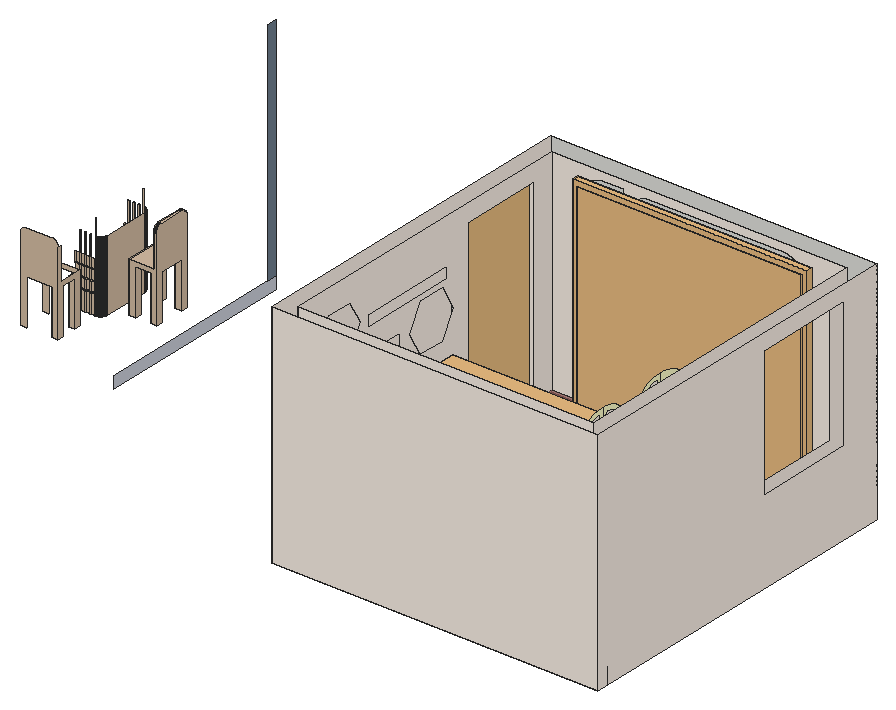
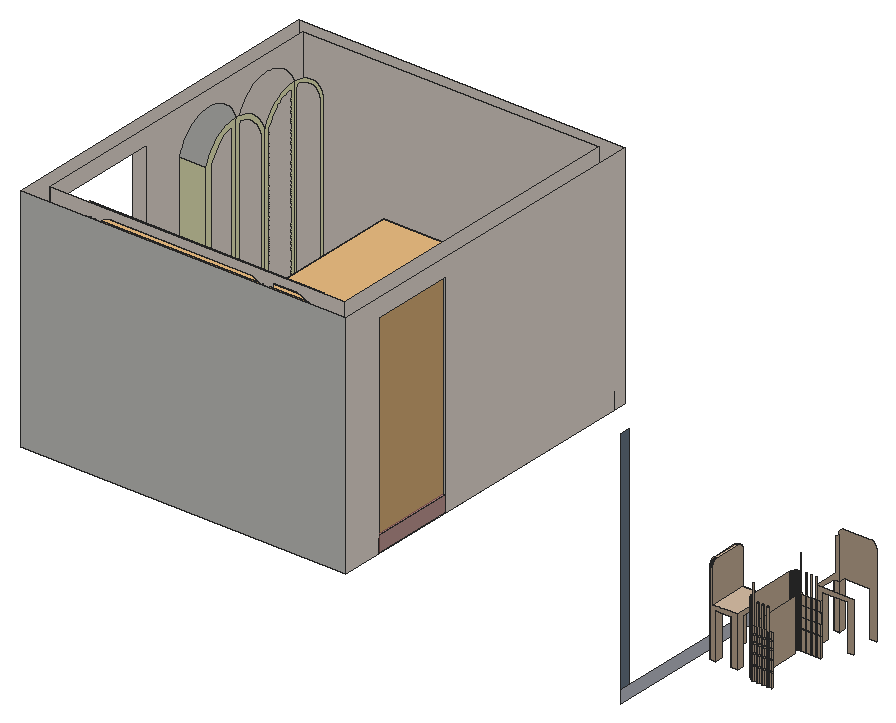
# SketchUp Ruby script. Lengths in inches.
U = 1.inch
M = Sketchup.active_model
def pt(a) = Geom::Point3d.new(a.map { |v| v * U })
def face(e, loops, mat)
  f = e.add_face(loops[0].map { |a| pt(a) })
  loops[1..].each { |l| e.add_face(l.map { |a| pt(a) }).erase! }
  f.material = f.back_material = mat if mat
  f
end
# faces: each face lists its corners as indices into pts; further lists are holes
def faces(e, pts, list, mat = nil) = list.each { |f| face(e, (f[0].is_a?(Array) ? f : [f]).map { |l| l.map { |i| pts[i] } }, mat) }
# xy, xz, yz: faces in a plane at the given z, y or x. An outline is a flat list of corners, or four numbers for a rectangle; further outlines are holes
def ring(l) = l.size == 4 ? [[l[0], l[1]], [l[2], l[1]], [l[2], l[3]], [l[0], l[3]]] : l.each_slice(2).to_a
def flat(e, list, mat, &to3) = list.each { |f| face(e, (f[0].is_a?(Array) ? f : [f]).map { |l| ring(l).map { |u, v| to3.(u, v) } }, mat) }
def xy(e, z, list, mat = nil) = flat(e, list, mat) { |x, y| [x, y, z] }
def xz(e, y, list, mat = nil) = flat(e, list, mat) { |x, z| [x, y, z] }
def yz(e, x, list, mat = nil) = flat(e, list, mat) { |y, z| [x, y, z] }
def lines(e, pts, list) = list.each { |a, b| e.add_line(pt(pts[a]), pt(pts[b])) }
# prism: a flat outline (further loops are holes) pulled along v
def prism(e, loops, v, mat = nil)
  f = face(e, loops, mat); d = Geom::Vector3d.new(v.map { |x| x * U })
  f.pushpull(f.normal.samedirection?(d) ? d.length : -d.length)
end
def box(e, o, s, mat = nil) = prism(e, [[o, [o[0] + s[0], o[1], o[2]], [o[0] + s[0], o[1] + s[1], o[2]], [o[0], o[1] + s[1], o[2]]]], [0, 0, s[2]], mat)
def at(x, y, z, deg = 0) = Geom::Transformation.translation(pt([x, y, z])) * Geom::Transformation.rotation(ORIGIN, Z_AXIS, deg.degrees)
def axes(o, x, y, z) = Geom::Transformation.new([*x, 0, *y, 0, *z, 0, *pt(o).to_a, 1])
def part(name) = M.definitions.add(name)
# library, detail: a bought-in or finely detailed component or shape, given as its bounding box
def library(name, o, s) = part(name).tap { |d| box(d.entities, o, s) }
def detail(e, o, s) = box(e.add_group.entities, o, s)
def put(e, d, t, mat = nil) = e.add_instance(d, t).tap { |i| i.material = mat if mat }
def group(e, t, mat = nil) = e.add_group.tap { |g| g.transformation = t; g.material = mat if mat }.entities
root = M.entities
M.materials.add("[0009_Linen]").color = [250, 240, 230]
M.materials.add("[0111_SlateGray]").color = [112, 128, 144]
M.materials.add("[Color E01]").color = [255, 255, 204]
M.materials.add("[Formica Laminate Light]").color = [213, 189, 164]
M.materials.add("[Marble Carrara Floor Tile]").color = [204, 208, 219]
M.materials.add("[Wood Square Tile 02]").color = [160, 101, 97]
M.materials["[Wood Square Tile 02]"].alpha = 0.73
c1 = library("1000x2100 L\#1",[0,0,0],[39.37,8.78,82.68])
c2 = library("Untitled+(2)",[-25.65,-58.99,0],[75.48,89.46,37.24])
xy(root,0,[[518.64,0,702.89,197]])
xy(root,0,[[315.45,97.95,319.1,101.59],[309.81,124.79,310.17,125.33],[312.73,124.79,313.09,125.33],[315.65,124.79,316.01,125.33],[318.58,124.79,318.9375,125.33],
  [309.52,159.08,310.35,159.77],[312.38,159.08,313.21,159.77],[315.25,159.08,316.07,159.77],[318.11,159.08,318.9375,159.77]],"[Formica Laminate Light]")
xy(root,7.64,[[307.48,159.08,309.52,159.77],[310.35,159.08,312.38,159.77],[313.21,159.08,315.25,159.77],[316.07,159.08,318.11,159.77]],"[Formica Laminate Light]")
xy(root,8.44,[[307.48,159.08,309.52,159.77],[310.35,159.08,312.38,159.77],[313.21,159.08,315.25,159.77],[316.07,159.08,318.11,159.77]],"[Formica Laminate Light]")
xy(root,9.25,[[527.89,6.9375,695.01,6.9375,695.01,12.1875,679.64,12.1875,679.64,94.5625,695.01,94.5625,695.01,185.9375,677.76,185.9375,677.76,179.1875,545.7,179.1875,545.7,185.9375,527.89,185.9375,527.89,173.6875,518.64,173.6875,518.64,126.5625,527.89,126.5625]],"[Wood Square Tile 02]")
xy(root,11.02,[[307.24,124.79,309.81,125.33],[310.17,124.79,312.73,125.33],[313.09,124.79,315.65,125.33],[316.01,124.79,318.58,125.33]],"[Formica Laminate Light]")
xy(root,11.55,[[307.24,124.79,309.81,125.33],[310.17,124.79,312.73,125.33],[313.09,124.79,315.65,125.33],[316.01,124.79,318.58,125.33]],"[Formica Laminate Light]")
xy(root,13.77,[[307.48,159.08,309.52,159.77],[310.35,159.08,312.38,159.77],[313.21,159.08,315.25,159.77],[316.07,159.08,318.11,159.77]],"[Formica Laminate Light]")
xy(root,14.57,[[307.48,159.08,309.52,159.77],[310.35,159.08,312.38,159.77],[313.21,159.08,315.25,159.77],[316.07,159.08,318.11,159.77]],"[Formica Laminate Light]")
xy(root,17.15,[[307.24,124.79,309.81,125.33],[310.17,124.79,312.73,125.33],[313.09,124.79,315.65,125.33],[316.01,124.79,318.58,125.33]],"[Formica Laminate Light]")
xy(root,19.01,[[307.48,159.08,309.52,159.77],[310.35,159.08,312.38,159.77],[313.21,159.08,315.25,159.77],[316.07,159.08,318.11,159.77]],"[Formica Laminate Light]")
xy(root,19.8125,[[307.48,159.08,309.52,159.77],[310.35,159.08,312.38,159.77],[313.21,159.08,315.25,159.77],[316.07,159.08,318.11,159.77]],"[Formica Laminate Light]")
xy(root,23.36,[[307.24,124.79,309.81,125.33],[310.17,124.79,312.73,125.33],[313.09,124.79,315.65,125.33],[316.01,124.79,318.58,125.33]],"[Formica Laminate Light]")
xy(root,23.54,[[307.48,159.08,309.52,159.77],[310.35,159.08,312.38,159.77],[313.21,159.08,315.25,159.77],[316.07,159.08,318.11,159.77]],"[Formica Laminate Light]")
xy(root,24.34,[[307.48,159.08,309.52,159.77],[310.35,159.08,312.38,159.77],[313.21,159.08,315.25,159.77],[316.07,159.08,318.11,159.77]],"[Formica Laminate Light]")
xy(root,28.25,[[329.76,134.98,343.65,156.18]],"[Formica Laminate Light]")
xy(root,50.4375,[[343.65,138.2,345.53,152.74]],"[Formica Laminate Light]")
xz(root,0,[[518.64,0,702.89,129.75]],"[0009_Linen]")
xz(root,6.9375,[[527.89,9.25,695.01,129.75]],"[0009_Linen]")
xz(root,12.1875,[[679.64,9.25,695.01,104.7]],"[Color E01]")
xz(root,53.375,[[679.64,9.25,695.01,104.7]])
xz(root,94.5625,[[679.64,9.25,695.01,104.7]],"[Color E01]")
xz(root,97.95,[[297.89,0,301.53,0,301.53,25.5625,315.45,25.5625,315.45,0,319.1,0,319.1,46.82,319.09,47.28,319.02,47.74,318.89,48.1875,318.7,48.61,318.45,49.01,318.15,49.37,317.8125,49.68,317.43,49.95,317.02,50.16,316.58,50.3125,316.125,50.41,315.66,50.4375,301.11,50.4375,300.68,50.36,300.26,50.23,299.85,50.05,299.47,49.82,299.125,49.55,298.8125,49.24,298.54,48.89,298.3125,48.52,298.13,48.12,298,47.69,297.92,47.26,297.89,46.82]],"[Formica Laminate Light]")
xz(root,101.59,[[315.45,0,319.1,25.5625]],"[Formica Laminate Light]")
xz(root,110.07,[[315.45,0,319.1,25.5625]],"[Formica Laminate Light]")
xz(root,113.72,[[297.89,0,297.89,28.25,319.1,28.25,319.1,0,315.45,0,315.45,25.5625,301.35,25.5625,301.35,0]],"[Formica Laminate Light]")
xz(root,124.79,[[309.81,0,310.17,40.33],[312.73,0,313.09,40.33],[315.65,0,316.01,40.33],[307.24,11.02,309.81,11.55],[310.17,11.02,312.73,11.55],
  [313.09,11.02,315.65,11.55],[316.01,11.02,318.58,11.55],[307.24,17.15,309.81,17.68],[310.17,17.15,312.73,17.68],[313.09,17.15,315.65,17.68],
  [316.01,17.15,318.58,17.68],[307.24,23.36,309.81,23.9],[310.17,23.36,312.73,23.9],[313.09,23.36,315.65,23.9],[316.01,23.36,318.58,23.9]],"[Formica Laminate Light]")
xz(root,125.33,[[307.24,0,309.81,11.02],[309.81,0,310.17,11.02],[310.17,0,312.73,11.02],[312.73,0,313.09,11.02],[313.09,0,315.65,11.02],
  [315.65,0,316.01,11.02],[316.01,0,318.58,11.02],[318.58,0,318.58,11.02,316.01,11.02,316.01,11.55,318.58,11.55,318.58,49.31,318.9375,49.31,318.9375,0],[309.81,11.02,310.17,11.55],[312.73,11.02,313.09,11.55],
  [315.65,11.02,316.01,11.55],[307.24,11.55,309.81,17.15],[309.81,11.55,310.17,40.33],[310.17,11.55,312.73,17.15],[312.73,11.55,313.09,40.33],
  [313.09,11.55,315.65,17.15],[315.65,11.55,316.01,40.33],[316.01,11.55,318.58,17.15],[307.24,17.15,309.81,23.36],[310.17,17.15,312.73,23.36],
  [313.09,17.15,315.65,23.36],[316.01,17.15,318.58,23.36],[307.24,23.36,309.81,28.96],[310.17,23.36,312.73,28.96],[313.09,23.36,315.65,28.96],
  [316.01,23.36,318.58,28.96]],"[Formica Laminate Light]")
xz(root,126.5625,[[518.64,9.25,527.89,119.9375]])
xz(root,134.98,[[329.76,0,333.4,0,333.4,25.5625,341.88,25.5625,341.88,0,345.53,0,345.53,46.82,343.65,46.82,343.65,28.25,329.76,28.25]],"[Formica Laminate Light]")
xz(root,138.43,[[329.76,0,333.4,25.5625]],"[Formica Laminate Light]")
xz(root,138.62,[[341.88,0,345.53,25.5625]],"[Formica Laminate Light]")
xz(root,152.54,[[329.76,0,333.4,25.5625],[341.88,0,345.53,25.5625]],"[Formica Laminate Light]")
xz(root,156.18,[[329.76,0,329.76,28.25,343.65,28.25,343.65,46.82,345.53,46.82,345.53,0,341.88,0,341.88,25.5625,333.4,25.5625,333.4,0]],"[Formica Laminate Light]")
xz(root,159.08,[[307.48,0,309.52,7.64],[309.52,0,310.35,40.33],[310.35,0,312.38,7.64],[312.38,0,313.21,40.33],[313.21,0,315.25,7.64],
  [315.25,0,316.07,40.33],[316.07,0,318.11,7.64],[318.11,0,318.9375,0,318.9375,49.31,318.11,49.31,318.11,8.44,316.07,8.44,316.07,7.64,318.11,7.64],[307.48,8.44,309.52,13.77],[310.35,8.44,312.38,13.77],
  [313.21,8.44,315.25,13.77],[316.07,8.44,318.11,13.77],[307.48,13.77,309.52,14.57],[310.35,13.77,312.38,14.57],[313.21,13.77,315.25,14.57],
  [316.07,13.77,318.11,14.57],[307.48,14.57,309.52,19.01],[310.35,14.57,312.38,19.01],[313.21,14.57,315.25,19.01],[316.07,14.57,318.11,19.01],
  [307.48,19.01,309.52,19.8125],[310.35,19.01,312.38,19.8125],[313.21,19.01,315.25,19.8125],[316.07,19.01,318.11,19.8125],[307.48,19.8125,309.52,23.54],
  [310.35,19.8125,312.38,23.54],[313.21,19.8125,315.25,23.54],[316.07,19.8125,318.11,23.54],[307.48,23.54,309.52,24.34],[310.35,23.54,312.38,24.34],
  [313.21,23.54,315.25,24.34],[316.07,23.54,318.11,24.34],[307.48,24.34,309.52,27.9],[310.35,24.34,312.38,27.9],[313.21,24.34,315.25,27.9],
  [316.07,24.34,318.11,27.9]],"[Formica Laminate Light]")
xz(root,159.77,[[309.52,0,310.35,40.33],[312.38,0,313.21,40.33],[315.25,0,316.07,40.33],[307.48,7.64,309.52,8.44],[310.35,7.64,312.38,8.44],
  [313.21,7.64,315.25,8.44],[316.07,7.64,318.11,8.44],[307.48,13.77,309.52,14.57],[310.35,13.77,312.38,14.57],[313.21,13.77,315.25,14.57],
  [316.07,13.77,318.11,14.57],[307.48,19.01,309.52,19.8125],[310.35,19.01,312.38,19.8125],[313.21,19.01,315.25,19.8125],[316.07,19.01,318.11,19.8125],
  [307.48,23.54,309.52,24.34],[310.35,23.54,312.38,24.34],[313.21,23.54,315.25,24.34],[316.07,23.54,318.11,24.34]],"[Formica Laminate Light]")
xz(root,173.6875,[[518.64,9.25,527.89,119.9375]],"[0009_Linen]")
xz(root,185.9375,[[[527.89,9.25,545.7,9.25,545.7,113.87,545.78,115.23,546.02,116.58,546.42,117.89,546.97,119.14,547.66,120.32,548.49,121.41,549.4375,122.39,550.5,123.25,551.65,123.99,552.89,124.58,554.18,125.02,555.52,125.3125,569.01,125.3125,569.01,47.68,569.08,46.64,569.28,45.61,569.62,44.62,570.08,43.68,570.66,42.8125,571.35,42.03,572.14,41.34,573.01,40.76,573.94,40.3,574.93,39.96,575.96,39.76,577,39.6875,659.67,39.6875,662.04,39.53,664.36,39.07,666.6,38.3125,668.72,37.26,670.68,35.95,672.46,34.39,674.02,32.61,675.34,30.64,676.38,28.52,677.14,26.28,677.61,23.96,677.76,21.6,677.76,9.25,695.01,9.25,695.01,129.75,527.89,129.75],[582.21,45.28,581.02,45.62,579.875,46.08,578.79,46.66,577.78,47.37,576.86,48.18,576.04,49.08,575.34,50.07,574.75,51.14,574.3,52.26,573.98,53.42,573.79,54.61,573.75,55.82,573.75,116.08,573.82,117.21,574.03,118.3125,574.375,119.39,574.85,120.41,575.46,121.375,576.17,122.26,576.99,123.05,577.91,123.75,578.9,124.33,579.96,124.78,581.07,125.11,582.21,125.3125,659.93,125.3125,661.12,125.23,662.29,124.99,663.4,124.58,664.45,124.03,665.41,123.34,666.25,122.53,666.97,121.61,667.55,120.6,667.97,119.52,668.24,118.39,668.26,118.12,668.33,117.24,668.26,116.08,668.26,55.82,668.19,54.63,667.99,53.46,667.66,52.3125,667.21,51.21,666.63,50.16,665.9375,49.18,665.14,48.28,664.25,47.46,663.27,46.75,662.21,46.14,661.1,45.65,659.93,45.28]]],"[0009_Linen]")
xz(root,197,[[518.64,0,702.89,129.75]])
yz(root,307.24,[[124.79,0,125.33,11.02],[124.79,11.02,125.33,11.55],[124.79,11.55,125.33,17.15],[124.79,23.36,125.33,28.96]],"[Formica Laminate Light]")
yz(root,307.48,[[159.08,0,159.77,7.64],[159.08,7.64,159.77,8.44],[159.08,8.44,159.77,13.77],[159.08,13.77,159.77,14.57],[159.08,14.57,159.77,19.01],
  [159.08,19.01,159.77,19.8125],[159.08,19.8125,159.77,23.54],[159.08,23.54,159.77,24.34],[159.08,24.34,159.77,27.9]],"[Formica Laminate Light]")
yz(root,309.52,[[159.08,0,159.77,7.64],[159.08,7.64,159.77,8.44],[159.08,8.44,159.77,13.77],[159.08,13.77,159.77,14.57],[159.08,14.57,159.77,19.01],
  [159.08,19.01,159.77,19.8125],[159.08,19.8125,159.77,23.54],[159.08,23.54,159.77,24.34],[159.08,24.34,159.77,27.9]],"[Formica Laminate Light]")
yz(root,309.81,[[124.79,0,125.33,11.02],[124.79,11.02,125.33,11.55],[124.79,11.55,125.33,17.15],[124.79,17.15,125.33,23.36],[124.79,23.36,125.33,28.96]],"[Formica Laminate Light]")
yz(root,310.17,[[124.79,0,125.33,11.02],[124.79,11.02,125.33,11.55],[124.79,11.55,125.33,17.15],[124.79,17.15,125.33,23.36],[124.79,23.36,125.33,28.96]],"[Formica Laminate Light]")
yz(root,310.35,[[159.08,0,159.77,7.64],[159.08,7.64,159.77,8.44],[159.08,8.44,159.77,13.77],[159.08,13.77,159.77,14.57],[159.08,14.57,159.77,19.01],
  [159.08,19.01,159.77,19.8125],[159.08,19.8125,159.77,23.54],[159.08,23.54,159.77,24.34],[159.08,24.34,159.77,27.9]],"[Formica Laminate Light]")
yz(root,312.38,[[159.08,0,159.77,7.64],[159.08,7.64,159.77,8.44],[159.08,8.44,159.77,13.77],[159.08,13.77,159.77,14.57],[159.08,14.57,159.77,19.01],
  [159.08,19.01,159.77,19.8125],[159.08,19.8125,159.77,23.54],[159.08,23.54,159.77,24.34],[159.08,24.34,159.77,27.9]],"[Formica Laminate Light]")
yz(root,312.73,[[124.79,0,125.33,11.02],[124.79,11.02,125.33,11.55],[124.79,11.55,125.33,17.15],[124.79,17.15,125.33,23.36],[124.79,23.36,125.33,28.96]],"[Formica Laminate Light]")
yz(root,313.09,[[124.79,0,125.33,11.02],[124.79,11.02,125.33,11.55],[124.79,11.55,125.33,17.15],[124.79,17.15,125.33,23.36],[124.79,23.36,125.33,28.96]],"[Formica Laminate Light]")
yz(root,313.21,[[159.08,0,159.77,7.64],[159.08,7.64,159.77,8.44],[159.08,8.44,159.77,13.77],[159.08,13.77,159.77,14.57],[159.08,14.57,159.77,19.01],
  [159.08,19.01,159.77,19.8125],[159.08,19.8125,159.77,23.54],[159.08,23.54,159.77,24.34],[159.08,24.34,159.77,27.9]],"[Formica Laminate Light]")
yz(root,315.25,[[159.08,0,159.77,7.64],[159.08,7.64,159.77,8.44],[159.08,8.44,159.77,13.77],[159.08,13.77,159.77,14.57],[159.08,14.57,159.77,19.01],
  [159.08,19.01,159.77,19.8125],[159.08,19.8125,159.77,23.54],[159.08,23.54,159.77,24.34],[159.08,24.34,159.77,27.9]],"[Formica Laminate Light]")
yz(root,315.45,[[97.95,0,101.59,25.5625],[110.07,0,113.72,25.5625]],"[Formica Laminate Light]")
yz(root,315.65,[[124.79,0,125.33,11.02],[124.79,11.02,125.33,11.55],[124.79,11.55,125.33,17.15],[124.79,17.15,125.33,23.36],[124.79,23.36,125.33,28.96]],"[Formica Laminate Light]")
yz(root,316.01,[[124.79,0,125.33,11.02],[124.79,11.02,125.33,11.55],[124.79,11.55,125.33,17.15],[124.79,17.15,125.33,23.36],[124.79,23.36,125.33,28.96]],"[Formica Laminate Light]")
yz(root,316.07,[[159.08,0,159.77,7.64],[159.08,7.64,159.77,8.44],[159.08,8.44,159.77,13.77],[159.08,13.77,159.77,14.57],[159.08,14.57,159.77,19.01],
  [159.08,19.01,159.77,19.8125],[159.08,19.8125,159.77,23.54],[159.08,23.54,159.77,24.34],[159.08,24.34,159.77,27.9]],"[Formica Laminate Light]")
yz(root,318.11,[[159.08,0,159.77,7.64],[159.08,8.44,159.77,13.77],[159.08,13.77,159.77,14.57],[159.08,14.57,159.77,19.01],[159.08,19.01,159.77,19.8125],
  [159.08,19.8125,159.77,23.54],[159.08,23.54,159.77,24.34],[159.08,24.34,159.77,27.9]],"[Formica Laminate Light]")
yz(root,318.58,[[124.79,0,125.33,11.02],[124.79,11.55,125.33,17.15],[124.79,17.15,125.33,23.36],[124.79,23.36,125.33,28.96]],"[Formica Laminate Light]")
yz(root,318.9375,[[128.96,0,155.08,28.69]],"[Formica Laminate Light]")
yz(root,319.1,[[97.95,0,101.59,0,101.59,25.5625,110.07,25.5625,110.07,0,113.72,0,113.72,28.25,99.82,28.25,99.82,46.82,97.95,46.82]],"[Formica Laminate Light]")
yz(root,322.35,[[128.96,0,155.08,40.33]],"[Formica Laminate Light]")
yz(root,329.76,[[134.98,0,134.98,28.25,156.18,28.25,156.18,0,152.54,0,152.54,25.5625,138.43,25.5625,138.43,0]],"[Formica Laminate Light]")
yz(root,333.4,[[134.98,0,138.43,25.5625],[152.54,0,156.18,25.5625]],"[Formica Laminate Light]")
yz(root,341.88,[[134.98,0,138.62,25.5625],[152.54,0,156.18,25.5625]],"[Formica Laminate Light]")
yz(root,343.65,[[134.98,28.25,134.98,46.82,135,47.26,135.08,47.69,135.21,48.12,135.4,48.52,135.625,48.89,135.9,49.24,136.21,49.55,136.56,49.82,136.9375,50.05,137.34,50.23,137.76,50.36,138.2,50.4375,152.74,50.4375,153.21,50.41,153.66,50.3125,154.1,50.16,154.52,49.95,154.9,49.68,155.24,49.37,155.54,49.01,155.78,48.61,155.97,48.1875,156.1,47.74,156.17,47.28,156.18,46.82,156.18,28.25]],"[Formica Laminate Light]")
yz(root,345.53,[[134.98,0,138.62,0,138.62,25.5625,152.54,25.5625,152.54,0,156.18,0,156.18,46.82,156.17,47.28,156.1,47.74,155.97,48.1875,155.78,48.61,155.54,49.01,155.24,49.37,154.9,49.68,154.52,49.95,154.1,50.16,153.66,50.3125,153.21,50.41,152.74,50.4375,138.2,50.4375,137.76,50.36,137.34,50.23,136.9375,50.05,136.56,49.82,136.21,49.55,135.9,49.24,135.625,48.89,135.4,48.52,135.21,48.12,135.08,47.69,135,47.26,134.98,46.82]],"[Formica Laminate Light]")
yz(root,358.53,[[197,0,202.625,129.75]],"[0111_SlateGray]")
yz(root,358.53,[[88,-6.9375,202.625,0]],"[Marble Carrara Floor Tile]")
yz(root,518.64,[[0,0,0,129.75,197,129.75,197,0,173.6875,0,173.6875,119.9375,126.5625,119.9375,126.5625,0]],"[0009_Linen]")
yz(root,518.64,[[126.5625,0,173.6875,9.25]],"[Wood Square Tile 02]")
yz(root,527.89,[[[6.9375,9.25,126.5625,9.25,126.5625,119.9375,173.6875,119.9375,173.6875,9.25,185.9375,9.25,185.9375,129.75,6.9375,129.75],[93.09,67.64,85.1875,81.33,93.09,95.02,108.9,95.02,116.8,81.33,108.9,67.64],[28.21,89.72,20.6,102.9,28.21,116.09,43.44,116.09,51.05,102.9,43.44,89.72],[24.59,78.19,78.67,85.38],[56.41,97.75,112.29,104.19]]],"[0009_Linen]")
yz(root,545.7,[[182.5625,9.25,185.9375,106.81]],"[Color E01]")
yz(root,677.76,[[182.5625,9.25,185.9375,21.6]],"[Color E01]")
yz(root,679.64,[[14.26,11.32,14.26,104.4,14.79,106.23,15.6,108.15,16.62,109.97,17.83,111.66,19.22,113.21,20.78,114.59,22.49,115.79,24.3125,116.8,26.24,117.59,28.24,118.16,30.29,118.51,30.29,11.32],[35.13,12.02,35.13,117.7,36.47,117.48,38.45,116.93,40.37,116.16,42.1875,115.19,43.89,114.04,45.46,112.7,46.88,111.2,48.12,109.56,49.18,107.79,50.04,105.92,50.6,104.25,50.6,12.02],[56.16,12.03,56.16,104.3,56.65,105.99,57.43,107.83,58.41,109.58,59.57,111.21,60.91,112.7,62.41,114.03,64.05,115.1875,65.81,116.15,67.66,116.92,69.59,117.47,70.78,117.67,70.78,12.03],[77.33,13.02,77.33,116.52,77.44,116.5,79.32,115.98,81.14,115.26,82.86,114.34,84.48,113.24,85.96,111.98,87.3,110.56,88.48,109,89.49,107.33,90.3,105.55,90.79,104.09,90.79,13.02]],"[0009_Linen]")
yz(root,679.64,[[[12.1875,9.25,12.1875,104.7,12.84,106.92,13.74,109.06,14.87,111.08,16.22,112.96,17.76,114.68,19.5,116.22,21.39,117.55,23.42,118.66,25.56,119.55,27.78,120.19,30.0625,120.57,32.36,120.7,32.36,9.25],[14.26,11.32,30.29,11.32,30.29,118.51,28.24,118.16,26.24,117.59,24.3125,116.8,22.49,115.79,20.78,114.59,19.22,113.21,17.83,111.66,16.62,109.97,15.6,108.15,14.79,106.23,14.26,104.4]],[[32.36,9.25,32.36,120.7,32.375,120.7,34.73,120.57,37.07,120.1875,39.34,119.56,41.54,118.68,43.62,117.57,45.58,116.24,47.375,114.71,49,113,50.42,111.11,51.64,109.09,52.625,106.94,53.375,104.7,53.375,9.25],[35.13,12.02,50.6,12.02,50.6,104.25,50.04,105.92,49.18,107.79,48.12,109.56,46.88,111.2,45.46,112.7,43.89,114.04,42.1875,115.19,40.37,116.16,38.45,116.93,36.47,117.48,35.13,117.7]],[[53.375,9.25,53.375,104.7,54.03,106.92,54.93,109.06,56.06,111.08,57.4,112.96,58.95,114.68,60.68,116.22,62.57,117.55,64.6,118.66,66.74,119.55,68.97,120.19,71.25,120.57,73.5625,120.7,73.5625,9.25],[56.16,12.03,70.78,12.03,70.78,117.67,69.59,117.47,67.66,116.92,65.81,116.15,64.05,115.1875,62.41,114.03,60.91,112.7,59.57,111.21,58.41,109.58,57.43,107.83,56.65,105.99,56.16,104.3]],[[73.5625,9.25,73.5625,120.7,75.92,120.57,78.25,120.1875,80.53,119.56,82.72,118.68,84.81,117.57,86.76,116.24,88.5625,114.71,90.18,113,91.61,111.11,92.83,109.09,93.8125,106.94,94.5625,104.7,94.5625,9.25],[77.33,13.02,90.79,13.02,90.79,104.09,90.3,105.55,89.49,107.33,88.48,109,87.3,110.56,85.96,111.98,84.48,113.24,82.86,114.34,81.14,115.26,79.32,115.98,77.44,116.5,77.33,116.52]]],"[Color E01]")
yz(root,695.01,[[53.375,9.25,53.375,104.7,54.03,106.92,54.93,109.06,56.06,111.08,57.4,112.96,58.95,114.68,60.68,116.22,62.57,117.55,64.6,118.66,66.74,119.55,68.97,120.19,71.25,120.57,73.5625,120.7,75.92,120.57,78.25,120.1875,80.53,119.56,82.72,118.68,84.81,117.57,86.76,116.24,88.5625,114.71,90.18,113,91.61,111.11,92.83,109.09,93.8125,106.94,94.5625,104.7,94.5625,9.25]])
yz(root,695.01,[[[6.9375,9.25,6.9375,129.75,185.9375,129.75,185.9375,9.25,94.5625,9.25,94.5625,104.7,93.8125,106.94,92.83,109.09,91.61,111.11,90.18,113,88.5625,114.71,86.76,116.24,84.81,117.57,82.72,118.68,80.53,119.56,78.25,120.1875,75.92,120.57,73.5625,120.7,71.25,120.57,68.97,120.19,66.74,119.55,64.6,118.66,62.57,117.55,60.68,116.22,58.95,114.68,57.4,112.96,56.06,111.08,54.93,109.06,54.03,106.92,53.375,104.7,52.625,106.94,51.64,109.09,50.42,111.11,49,113,47.375,114.71,45.58,116.24,43.62,117.57,41.54,118.68,39.34,119.56,37.07,120.1875,34.73,120.57,32.375,120.7,30.0625,120.57,27.78,120.19,25.56,119.55,23.42,118.66,21.39,117.55,19.5,116.22,17.76,114.68,16.22,112.96,14.87,111.08,13.74,109.06,12.84,106.92,12.1875,104.7,12.1875,9.25],[117.4375,47.26,174.3125,120.7]]],"[0009_Linen]")
yz(root,702.89,[[[0,0,197,129.75],[117.4375,47.26,174.3125,120.7]]],"[0009_Linen]")
p = [[318.9375,125.33,40.33],[318.9375,125.33,0],[319.39,125.38,0],[319.39,125.38,40.33],[319.84,125.5,0],[319.84,125.5,40.33],
  [320.26,125.67,0],[320.26,125.67,40.33],[320.66,125.89,0],[320.66,125.89,40.33],[321.03,126.16,0],[321.03,126.16,40.33],
  [321.37,126.47,0],[321.37,126.47,40.33],[321.66,126.82,0],[321.66,126.82,40.33],[321.9,127.21,0],[321.9,127.21,40.33],
  [322.1,127.62,0],[322.1,127.62,40.33],[322.24,128.06,0],[322.24,128.06,40.33],[322.33,128.51,0],[322.33,128.51,40.33],
  [322.35,128.96,0],[322.35,128.96,40.33],[322.35,155.08,40.33],[322.35,155.08,0],[322.33,155.56,0],[322.33,155.56,40.33],
  [322.24,156.03,0],[322.24,156.03,40.33],[322.1,156.48,0],[322.1,156.48,40.33],[321.91,156.92,0],[321.91,156.92,40.33],
  [321.67,157.33,0],[321.67,157.33,40.33],[321.38,157.71,0],[321.38,157.71,40.33],[321.05,158.05,0],[321.05,158.05,40.33],
  [320.69,158.36,0],[320.69,158.36,40.33],[320.28,158.62,0],[320.28,158.62,40.33],[319.85,158.82,0],[319.85,158.82,40.33],
  [319.4,158.98,0],[319.4,158.98,40.33],[318.9375,159.08,0],[318.9375,159.08,40.33],[677.61,185.9375,23.96],[677.61,182.5625,23.96],
  [677.76,182.5625,21.6],[677.76,185.9375,21.6],[677.14,185.9375,26.28],[677.14,182.5625,26.28],[343.65,135,47.26],[343.65,134.98,46.82],
  [345.53,134.98,46.82],[345.53,135,47.26],[343.65,156.18,46.82],[343.65,156.17,47.28],[345.53,156.17,47.28],[345.53,156.18,46.82],
  [343.65,135.08,47.69],[345.53,135.08,47.69],[343.65,156.1,47.74],[345.53,156.1,47.74],[343.65,135.21,48.12],[345.53,135.21,48.12],
  [343.65,155.97,48.1875],[345.53,155.97,48.1875],[343.65,135.4,48.52],[345.53,135.4,48.52],[343.65,155.78,48.61],[345.53,155.78,48.61],
  [343.65,135.625,48.89],[345.53,135.625,48.89],[343.65,155.54,49.01],[345.53,155.54,49.01],[343.65,135.9,49.24],[345.53,135.9,49.24],
  [343.65,155.24,49.37],[345.53,155.24,49.37],[343.65,136.21,49.55],[345.53,136.21,49.55],[343.65,154.9,49.68],[345.53,154.9,49.68],
  [343.65,136.56,49.82],[345.53,136.56,49.82],[343.65,154.52,49.95],[345.53,154.52,49.95],[343.65,136.9375,50.05],[345.53,136.9375,50.05],
  [343.65,154.1,50.16],[345.53,154.1,50.16],[343.65,137.34,50.23],[345.53,137.34,50.23],[343.65,137.76,50.36],[345.53,137.76,50.36],
  [343.65,153.66,50.3125],[345.53,153.66,50.3125],[343.65,153.21,50.41],[345.53,153.21,50.41],[343.65,138.2,50.4375],[345.53,138.2,50.4375],
  [343.65,152.74,50.4375],[345.53,152.74,50.4375],[318.9375,124.79,0],[318.9375,124.79,40.33],[318.9375,159.77,0],[318.9375,159.77,40.33],
  [702.89,6.9375,0],[702.89,6.9375,9.25],[518.64,6.9375,0],[518.64,6.9375,9.25],[527.89,6.9375,9.25],[695.01,6.9375,9.25]]
faces(root,p,[[0,1,2,3],[3,2,4,5],[5,4,6,7],[7,6,8,9],[9,8,10,11],[11,10,12,13],[13,12,14,15],[15,14,16,17],
  [17,16,18,19],[19,18,20,21],[21,20,22,23],[23,22,24,25],[26,27,28,29],[29,28,30,31],[31,30,32,33],[33,32,34,35],
  [35,34,36,37],[37,36,38,39],[39,38,40,41],[41,40,42,43],[43,42,44,45],[45,44,46,47],[47,46,48,49],[49,48,50,51],
  [58,59,60,61],[62,63,64,65],[66,58,61,67],[63,68,69,64],[70,66,67,71],[68,72,73,69],[74,70,71,75],[72,76,77,73],
  [78,74,75,79],[76,80,81,77],[82,78,79,83],[80,84,85,81],[86,82,83,87],[84,88,89,85],[90,86,87,91],[88,92,93,89],
  [94,90,91,95],[92,96,97,93],[98,94,95,99],[100,98,99,101],[96,102,103,97],[102,104,105,103],[106,100,101,107],[104,108,109,105]],"[Formica Laminate Light]")
faces(root,p,[[52,53,54,55],[56,57,53,52]],"[Color E01]")
lines(root,p,[[110,111],[112,113],[114,115],[116,117],[118,117],[119,115]])
detail(root,[548.56,178.4375,12.11],[126.34,7.5,110.34])
put(root,c1,axes([520.1,173.6875,9.25],[0,-1.19697,0],[0.58,0,0],[0,0,1.33879]))
put(root,c2,axes([567.93,52.22,9.25],[0,1.18,0],[-1.18,0,0],[0,0,1.4042]))
g1 = group(root,at(545.7,179.1875,9.25))
p = [[0,3.375,0],[132.0625,3.375,0]]
lines(g1,p,[[0,1]])
detail(g1,[0,0,0],[132.0625,3.375,116.0625])
